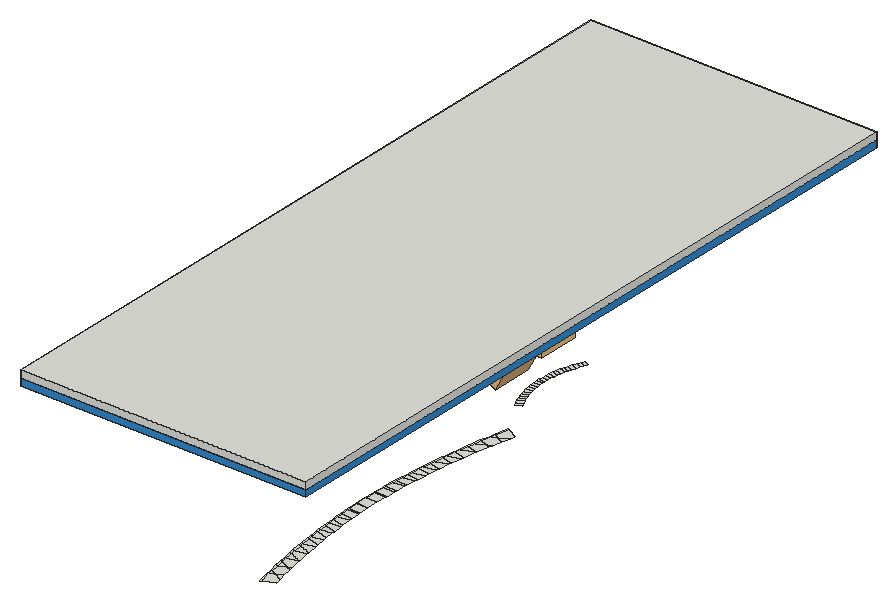
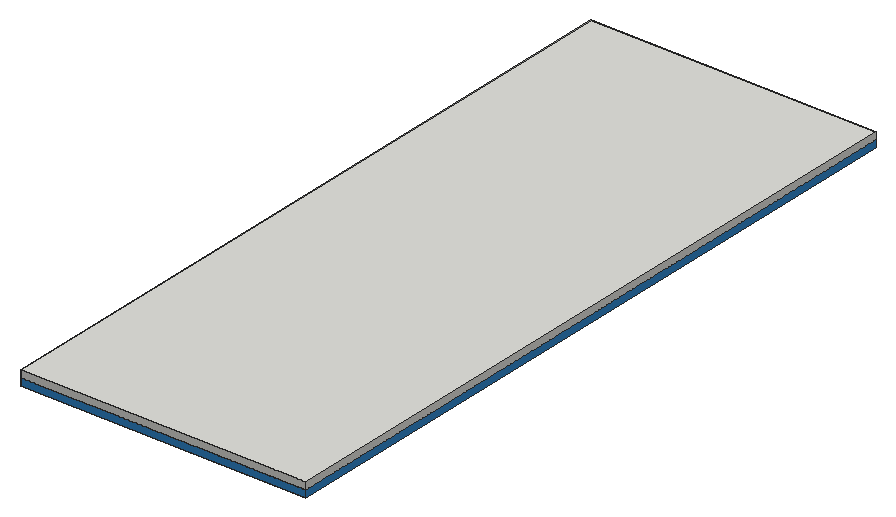
# SketchUp Ruby script. Lengths in inches.
U = 1.inch
M = Sketchup.active_model
def pt(a) = Geom::Point3d.new(a.map { |v| v * U })
def face(e, loops, mat)
  f = e.add_face(loops[0].map { |a| pt(a) })
  loops[1..].each { |l| e.add_face(l.map { |a| pt(a) }).erase! }
  f.material = f.back_material = mat if mat
  f
end
# faces: each face lists its corners as indices into pts; further lists are holes
def faces(e, pts, list, mat = nil) = list.each { |f| face(e, (f[0].is_a?(Array) ? f : [f]).map { |l| l.map { |i| pts[i] } }, mat) }
# xy, xz, yz: faces in a plane at the given z, y or x. An outline is a flat list of corners, or four numbers for a rectangle; further outlines are holes
def ring(l) = l.size == 4 ? [[l[0], l[1]], [l[2], l[1]], [l[2], l[3]], [l[0], l[3]]] : l.each_slice(2).to_a
def flat(e, list, mat, &to3) = list.each { |f| face(e, (f[0].is_a?(Array) ? f : [f]).map { |l| ring(l).map { |u, v| to3.(u, v) } }, mat) }
def xy(e, z, list, mat = nil) = flat(e, list, mat) { |x, y| [x, y, z] }
def xz(e, y, list, mat = nil) = flat(e, list, mat) { |x, z| [x, y, z] }
def yz(e, x, list, mat = nil) = flat(e, list, mat) { |y, z| [x, y, z] }
def lines(e, pts, list) = list.each { |a, b| e.add_line(pt(pts[a]), pt(pts[b])) }
# prism: a flat outline (further loops are holes) pulled along v
def prism(e, loops, v, mat = nil)
  f = face(e, loops, mat); d = Geom::Vector3d.new(v.map { |x| x * U })
  f.pushpull(f.normal.samedirection?(d) ? d.length : -d.length)
end
def box(e, o, s, mat = nil) = prism(e, [[o, [o[0] + s[0], o[1], o[2]], [o[0] + s[0], o[1] + s[1], o[2]], [o[0], o[1] + s[1], o[2]]]], [0, 0, s[2]], mat)
def at(x, y, z, deg = 0) = Geom::Transformation.translation(pt([x, y, z])) * Geom::Transformation.rotation(ORIGIN, Z_AXIS, deg.degrees)
def axes(o, x, y, z) = Geom::Transformation.new([*x, 0, *y, 0, *z, 0, *pt(o).to_a, 1])
def part(name) = M.definitions.add(name)
# library, detail: a bought-in or finely detailed component or shape, given as its bounding box
def library(name, o, s) = part(name).tap { |d| box(d.entities, o, s) }
def detail(e, o, s) = box(e.add_group.entities, o, s)
def put(e, d, t, mat = nil) = e.add_instance(d, t).tap { |i| i.material = mat if mat }
def group(e, t, mat = nil) = e.add_group.tap { |g| g.transformation = t; g.material = mat if mat }.entities
root = M.entities
M.materials.add("Emissive").color = [255, 255, 255]
M.materials.add("[Color I07]").color = [53, 140, 209]
c1 = library("dolphin",[-25.31,-46.61,-0.13],[46.1,106.17,73.53])
c2 = part("Group\#18")
xy(c2.entities,0,[[12.88,0,16.04,8.74,18.67,17.76,20.72,26.92,22.19,36.19,23.08,45.54,23.375,54.93,23.08,64.31,22.19,73.66,20.72,82.93,18.67,92.09,16.04,101.11,12.92,109.75,9.91,120.33,7.43,131.07,5.5,141.93,4.11,152.87,3.28,163.86,3,174.88,3.28,185.9,4.11,196.9,5.5,207.84,7.43,218.69,9.91,229.44,12.95,240.11,10.0625,240.93,7,230.18,4.49,219.29,2.53,208.29,1.125,197.2,0.28,186.06,0,174.88,0.28,163.71,1.125,152.5625,2.53,141.48,4.49,130.47,7,119.58,10.0625,108.83,13.1875,100.18,15.76,91.34,17.77,82.37,19.22,73.28,20.09,64.12,20.375,54.93,20.09,45.73,19.22,36.57,17.77,27.48,15.76,18.51,13.1875,9.67,10.0625,1.02]])
xy(root,44,[[201.82,0,202.8,0.22,200.26,11.66,199.28,11.47],[202.8,0.22,212.15,4.84,211.37,8.47,203.64,12.99,200.26,11.66],[211.37,8.47,209.51,15.61,203.64,12.99],[199.28,11.47,200.26,11.66,199.65,15.33,198.66,15.15],[200.26,11.66,203.64,12.99,199.65,15.33],
  [203.64,12.99,209.51,15.61,207.95,23.33,204.28,25.25,198.01,23.07,199.65,15.33],[198.66,15.15,199.65,15.33,198.01,23.07,197.03,22.89],[197.03,22.89,198.01,23.07,197.09,29.01,196.1,28.84],[198.01,23.07,204.28,25.25,197.09,29.01],[207.95,23.33,207.19,26.4,204.28,25.25],
  [204.28,25.25,207.19,26.4,205.21,36.84,204.76,37.05,196,34.4,197.09,29.01],[196.1,28.84,197.09,29.01,196,34.4,195.01,34.23],[195.01,34.23,196,34.4,194.97,41.57,193.99,41.41],[196,34.4,204.76,37.05,194.97,41.57],[205.21,36.84,205.13,37.17,204.76,37.05],
  [204.76,37.05,205.13,37.17,203.24,47.92,194.2,45.63,194.97,41.57],[193.99,41.41,194.97,41.57,194.2,45.63,193.21,45.47],[193.21,45.47,194.2,45.63,193.2,53.25,192.21,53.1],[194.2,45.63,203.24,47.92,203.09,49.24,193.2,53.25],[203.09,49.24,201.57,58.57,192.58,56.72,193.2,53.25],
  [192.21,53.1,193.2,53.25,192.58,56.72,191.59,56.57],[191.59,56.57,192.58,56.72,191.71,64.21,190.72,64.07],[192.58,56.72,201.57,58.57,201.35,60.83,191.71,64.21],[201.35,60.83,200.12,69.11,191.15,67.64,191.71,64.21],[190.72,64.07,191.71,64.21,191.15,67.64,190.16,67.51],
  [190.16,67.51,191.15,67.64,190.46,74.59,189.47,74.47],[191.15,67.64,200.12,69.11,199.89,71.79,190.46,74.59],[199.89,71.79,198.87,79.53,189.91,78.39,190.46,74.59],[189.47,74.47,190.46,74.59,189.91,78.39,188.91,78.28],[188.91,78.28,189.91,78.39,189.43,84.51,188.44,84.41],
  [189.91,78.39,198.87,79.53,198.7,82.24,189.43,84.51],[198.7,82.24,197.84,89.82,188.86,88.98,189.43,84.51],[188.44,84.41,189.43,84.51,188.86,88.98,187.87,88.89],[187.87,88.89,188.86,88.98,188.59,94.0625,187.59,93.99],[188.86,88.98,197.84,89.82,197.74,92.28,188.59,94.0625],
  [197.74,92.28,197.03,100.01,188.04,99.42,188.59,94.0625],[187.59,93.99,188.59,94.0625,188.04,99.42,187.04,99.35],[187.04,99.35,188.04,99.42,187.93,103.33,186.94,103.28],[188.04,99.42,197.03,100.01,197,102.01,187.93,103.33],[197,102.01,196.45,110.11,187.45,109.73,187.93,103.33],
  [186.94,103.28,187.93,103.33,187.45,109.73,186.45,109.7],[186.45,109.7,187.45,109.73,187.45,112.39,186.45,112.36],[187.45,109.73,196.45,110.11,196.46,111.52,187.45,112.39],[196.46,111.52,196.11,120.15,187.1,119.96,187.45,112.39],[186.45,112.36,187.45,112.39,187.1,119.96,186.1,119.96],
  [186.1,119.96,187.1,119.96,187.15,121.31,186.15,121.3125],[187.1,119.96,196.11,120.15,196.13,120.87,187.15,121.31],[196.13,120.87,196.01,130.15,187.01,130.15,187.15,121.31],[187.15,121.31,187.01,130.15,186.01,130.15,186.15,121.3125],[186.01,130.15,187.01,130.15,187.15,139,186.15,138.99],
  [187.01,130.15,196.01,130.15,196.13,139.43,187.15,139],[186.15,138.99,187.15,139,187.1,140.34,186.1,140.35],[187.15,139,196.13,139.43,196.11,140.16,187.1,140.34],[196.11,140.16,196.46,148.79,187.45,147.92,187.1,140.34],[187.1,140.34,187.45,147.92,186.45,147.94,186.1,140.35],
  [187.45,147.92,187.45,150.57,186.45,150.61,186.45,147.94],[187.45,147.92,196.46,148.79,196.45,150.19,187.45,150.57],[196.45,150.19,197,158.29,187.93,156.98,187.45,150.57],[187.45,150.57,187.93,156.98,186.94,157.03,186.45,150.61],[187.93,156.98,188.04,160.89,187.04,160.95,186.94,157.03],
  [187.93,156.98,197,158.29,197.03,160.29,188.04,160.89],[197.03,160.29,197.74,168.03,188.59,166.24,188.04,160.89],[188.04,160.89,188.59,166.24,187.59,166.32,187.04,160.95],[188.59,166.24,188.86,171.33,187.87,171.42,187.59,166.32],[188.59,166.24,197.74,168.03,197.84,170.48,188.86,171.33],
  [197.84,170.48,198.7,178.07,189.43,175.79,188.86,171.33],[188.86,171.33,189.43,175.79,188.44,175.89,187.87,171.42],[189.43,175.79,189.91,181.91,188.91,182.03,188.44,175.89],[189.43,175.79,198.7,178.07,198.87,180.78,189.91,181.91],[198.87,180.78,199.89,188.52,190.46,185.71,189.91,181.91],
  [189.91,181.91,190.46,185.71,189.47,185.83,188.91,182.03],[190.46,185.71,191.15,192.67,190.16,192.8,189.47,185.83],[190.46,185.71,199.89,188.52,200.12,191.2,191.15,192.67],[200.12,191.2,201.35,199.47,191.71,196.1,191.15,192.67],[191.15,192.67,191.71,196.1,190.72,196.23,190.16,192.8],
  [191.71,196.1,192.58,203.59,191.59,203.74,190.72,196.23],[191.71,196.1,201.35,199.47,201.57,201.74,192.58,203.59],[201.57,201.74,203.09,211.07,193.2,207.06,192.58,203.59],[192.58,203.59,193.2,207.06,192.21,207.21,191.59,203.74],[193.2,207.06,194.2,214.68,193.21,214.83,192.21,207.21],
  [193.2,207.06,203.09,211.07,203.24,212.39,194.2,214.68],[203.24,212.39,205.13,223.13,204.76,223.26,194.97,218.73,194.2,214.68],[194.2,214.68,194.97,218.73,193.99,218.9,193.21,214.83],[194.97,218.73,196,225.9,195.01,226.07,193.99,218.9],[194.97,218.73,204.76,223.26,196,225.9],
  [205.13,223.13,205.21,223.47,204.76,223.26],[204.76,223.26,205.21,223.47,207.19,233.91,204.28,235.05,197.09,231.29,196,225.9],[196,225.9,197.09,231.29,196.1,231.47,195.01,226.07],[197.09,231.29,198.01,237.24,197.03,237.42,196.1,231.47],[197.09,231.29,204.28,235.05,198.01,237.24],
  [207.19,233.91,207.95,236.97,204.28,235.05],[204.28,235.05,207.95,236.97,209.51,244.7,203.64,247.3125,199.65,244.98,198.01,237.24],[198.01,237.24,199.65,244.98,198.66,245.16,197.03,237.42],[209.51,244.7,211.37,251.84,203.64,247.3125],[199.65,244.98,200.26,248.65,199.28,248.84,198.66,245.16],
  [199.65,244.98,203.64,247.3125,200.26,248.65],[203.64,247.3125,211.37,251.84,212.15,255.46,202.8,260.09,200.26,248.65],[200.26,248.65,202.8,260.09,201.82,260.31,199.28,248.84],[185.34,288.6,186.23,289.04,189.78,290.89,188.44,293.58,183.92,291.45],[183.92,291.45,188.44,293.58,187.22,296.32,182.61,294.37],
  [182.61,294.37,187.22,296.32,186.1,299.1,181.42,297.34],[181.42,297.34,186.1,299.1,185.1,301.93,180.36,300.35],[180.36,300.35,185.1,301.93,184.21,304.8,179.41,303.41],[179.41,303.41,184.21,304.8,183.44,307.69,178.58,306.5],[178.58,306.5,183.44,307.69,182.78,310.62,177.88,309.625],
  [177.88,309.625,182.78,310.62,182.25,313.57,177.31,312.77],[177.31,312.77,182.25,313.57,181.83,316.54,176.86,315.94],[176.86,315.94,181.83,316.54,181.53,319.53,176.54,319.13],[176.54,319.13,181.53,319.53,181.35,322.52,176.35,322.32],[176.35,322.32,181.35,322.52,181.29,325.52,176.29,325.52],
  [176.29,325.52,181.29,325.52,181.35,328.52,176.35,328.72],[181.35,328.52,181.53,331.52,176.54,331.92,176.35,328.72],[181.53,331.52,181.83,334.5,176.86,335.1,176.54,331.92],[181.83,334.5,182.25,337.47,177.31,338.27,176.86,335.1],[182.25,337.47,182.78,340.42,177.88,341.42,177.31,338.27],
  [182.78,340.42,183.44,343.35,178.58,344.54,177.88,341.42],[183.44,343.35,184.21,346.25,179.41,347.63,178.58,344.54],[184.21,346.25,185.1,349.11,180.36,350.6875,179.41,347.63],[185.1,349.11,186.1,351.94,181.42,353.7,180.36,350.6875],[186.1,351.94,187.22,354.72,182.61,356.68,181.42,353.7],
  [187.22,354.72,188.44,357.46,183.92,359.6,182.61,356.68],[188.44,357.46,189.78,360.15,186.23,362,185.34,362.44,183.92,359.6]])
put(root,c1,axes([168.05,299.6875,59.47],[-0.28974,-0.0064,0.15782],[0.00729,-0.32992,0],[0.15778,0.00349,0.28982]))
put(root,c1,axes([178.75,331.67,67.4375],[0.33,0,0],[0,0.33,0],[0,0,0.33]))
put(root,c2,at(41.91,44.17,120.1875),"Emissive")
put(root,c2,axes([198.09,44.17,120.1875],[-1,0,0],[0,1,0],[0,0,1]),"Emissive")
g1 = group(root,at(0,0.22,120.1875),"[Color I07]")
box(g1,[0,0,0],[240,600,6])
g2 = group(root,at(0,0.22,126.1875))
box(g2,[0,0,0],[240,600,6])
